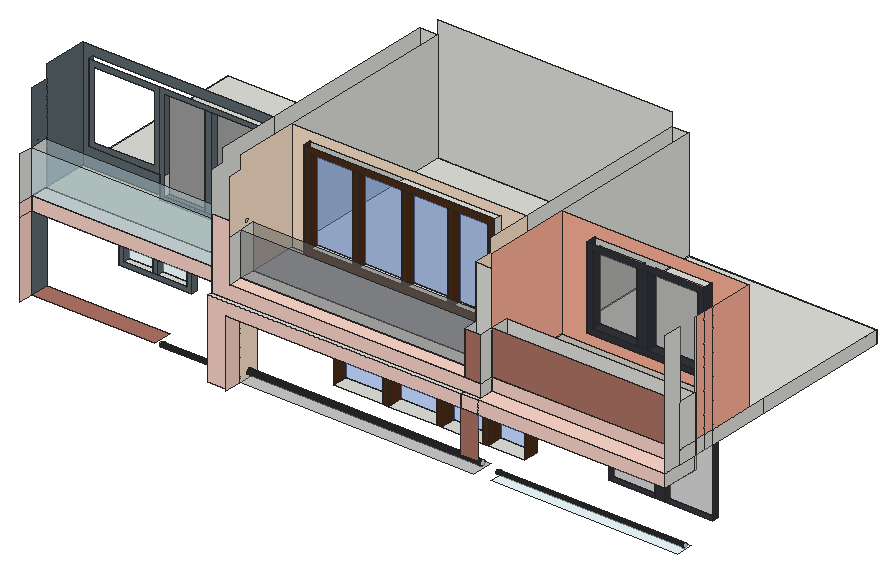
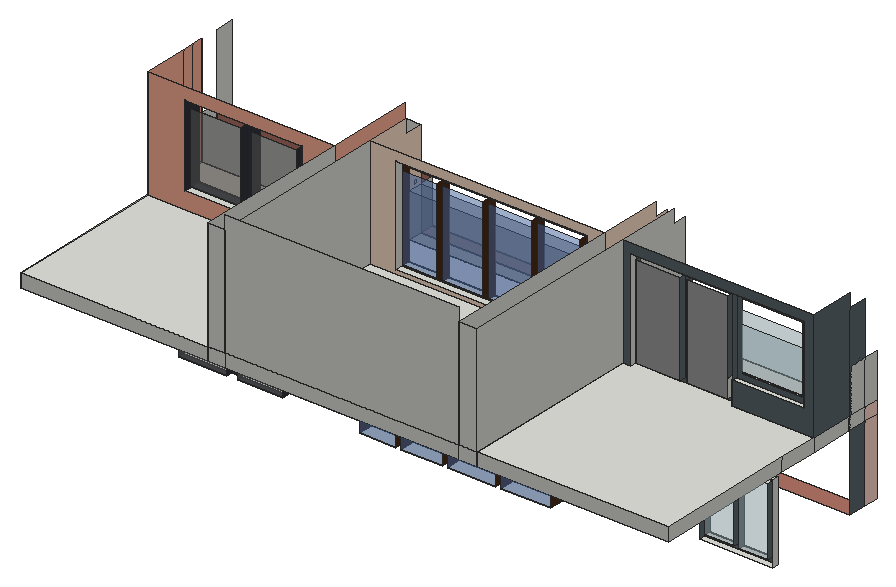
# SketchUp Ruby script. Lengths in inches.
U = 1.inch
M = Sketchup.active_model
def pt(a) = Geom::Point3d.new(a.map { |v| v * U })
def face(e, loops, mat)
  f = e.add_face(loops[0].map { |a| pt(a) })
  loops[1..].each { |l| e.add_face(l.map { |a| pt(a) }).erase! }
  f.material = f.back_material = mat if mat
  f
end
# faces: each face lists its corners as indices into pts; further lists are holes
def faces(e, pts, list, mat = nil) = list.each { |f| face(e, (f[0].is_a?(Array) ? f : [f]).map { |l| l.map { |i| pts[i] } }, mat) }
# xy, xz, yz: faces in a plane at the given z, y or x. An outline is a flat list of corners, or four numbers for a rectangle; further outlines are holes
def ring(l) = l.size == 4 ? [[l[0], l[1]], [l[2], l[1]], [l[2], l[3]], [l[0], l[3]]] : l.each_slice(2).to_a
def flat(e, list, mat, &to3) = list.each { |f| face(e, (f[0].is_a?(Array) ? f : [f]).map { |l| ring(l).map { |u, v| to3.(u, v) } }, mat) }
def xy(e, z, list, mat = nil) = flat(e, list, mat) { |x, y| [x, y, z] }
def xz(e, y, list, mat = nil) = flat(e, list, mat) { |x, z| [x, y, z] }
def yz(e, x, list, mat = nil) = flat(e, list, mat) { |y, z| [x, y, z] }
def lines(e, pts, list) = list.each { |a, b| e.add_line(pt(pts[a]), pt(pts[b])) }
# prism: a flat outline (further loops are holes) pulled along v
def prism(e, loops, v, mat = nil)
  f = face(e, loops, mat); d = Geom::Vector3d.new(v.map { |x| x * U })
  f.pushpull(f.normal.samedirection?(d) ? d.length : -d.length)
end
def box(e, o, s, mat = nil) = prism(e, [[o, [o[0] + s[0], o[1], o[2]], [o[0] + s[0], o[1] + s[1], o[2]], [o[0], o[1] + s[1], o[2]]]], [0, 0, s[2]], mat)
def at(x, y, z, deg = 0) = Geom::Transformation.translation(pt([x, y, z])) * Geom::Transformation.rotation(ORIGIN, Z_AXIS, deg.degrees)
def axes(o, x, y, z) = Geom::Transformation.new([*x, 0, *y, 0, *z, 0, *pt(o).to_a, 1])
def part(name) = M.definitions.add(name)
# library, detail: a bought-in or finely detailed component or shape, given as its bounding box
def library(name, o, s) = part(name).tap { |d| box(d.entities, o, s) }
def detail(e, o, s) = box(e.add_group.entities, o, s)
def put(e, d, t, mat = nil) = e.add_instance(d, t).tap { |i| i.material = mat if mat }
def group(e, t, mat = nil) = e.add_group.tap { |g| g.transformation = t; g.material = mat if mat }.entities
root = M.entities
M.materials.add("[Blinds Vertical Stripe Gray]").color = [160, 160, 160]
M.materials.add("[Color B01]").color = [255, 216, 204]
M.materials.add("[Color B02]").color = [255, 178, 153]
M.materials.add("[Color C01]").color = [255, 229, 204]
M.materials.add("[Field Rectangle Tile]").color = [196, 189, 179]
M.materials.add("[Field Square Tile]").color = [217, 201, 169]
M.materials.add("[Formica Graystone]").color = [149, 146, 135]
M.materials.add("[Formica Laminate Dark]").color = [50, 53, 60]
M.materials.add("[Formica Speckled Grey]").color = [94, 105, 111]
M.materials.add("[Marble Carrara Floor Tile]").color = [204, 208, 219]
M.materials.add("[Stone Flagstone Ashlar]").color = [175, 116, 102]
M.materials.add("[Stone Flagstone Ashlar]1").color = [175, 116, 102]
M.materials.add("[Terrazzo Tile Light]").color = [219, 217, 210]
M.materials.add("[Translucent Glass Blue]").color = [100, 149, 237]
M.materials["[Translucent Glass Blue]"].alpha = 0.5
M.materials.add("[Translucent Glass Gray]").color = [128, 128, 128]
M.materials["[Translucent Glass Gray]"].alpha = 0.5
M.materials.add("[Translucent Glass Safety]").color = [204, 235, 244]
M.materials["[Translucent Glass Safety]"].alpha = 0.5
M.materials.add("[Wood Veneer 01]").color = [76, 44, 23]
xy(root,776.18,[[1324.98,1141.09,1459.45,1182.72],[1473.64,1141.09,1605.14,1182.72],[1619.33,1141.09,1732.89,1182.72],[1747.08,1141.09,1847.2,1182.72]])
xy(root,789.44,[[2056.09,1166.78,2180.58,1182.72],[2208.79,1166.78,2341.44,1182.72]],"[Formica Laminate Dark]")
xy(root,844.43,[[715.78,1166.28,917.47,1182.72]])
xy(root,858.1,[[729.45,1166.28,809.37,1182.72],[823.58,1166.28,903.8,1182.72]])
xy(root,868.4375,[[1131.83,916.51,1132.91,916.65,1133.92,917.07,1134.79,917.73,1135.46,918.6,1135.875,919.61,1136.02,920.69,1135.875,921.78,1135.46,922.79,1134.79,923.65,1133.92,924.32,1132.91,924.74,1131.83,924.88,1130.75,924.74,1129.74,924.32,1128.87,923.65,1128.2,922.79,1127.79,921.78,1127.64,920.69,1127.79,919.61,1128.2,918.6,1128.87,917.73,1129.74,917.07,1130.75,916.65]])
xy(root,868.4375,[[1263.92,894.5,1905.54,954.56]],"[Translucent Glass Gray]")
xy(root,868.4375,[[1950.59,894.5,2463.34,942.43]],"[Translucent Glass Safety]")
xy(root,868.5625,[[1101.58,916.51,1102.66,916.65,1103.67,917.07,1104.54,917.73,1105.21,918.6,1105.625,919.61,1105.77,920.69,1105.625,921.78,1105.21,922.79,1104.54,923.65,1103.67,924.32,1102.66,924.74,1101.58,924.88,1100.5,924.74,1099.49,924.32,1098.62,923.65,1097.95,922.79,1097.54,921.78,1097.39,920.69,1097.54,919.61,1097.95,918.6,1098.62,917.73,1099.49,917.07,1100.5,916.65]])
xy(root,868.875,[[1167.14,916.51,1168.23,916.65,1169.24,917.07,1170.1,917.73,1170.77,918.6,1171.1875,919.61,1171.33,920.69,1171.1875,921.78,1170.77,922.79,1170.1,923.65,1169.24,924.32,1168.23,924.74,1167.14,924.88,1166.06,924.74,1165.05,924.32,1164.18,923.65,1163.52,922.79,1163.1,921.78,1162.96,920.69,1163.1,919.61,1163.52,918.6,1164.18,917.73,1165.05,917.07,1166.06,916.65]])
xy(root,869.875,[[1198.52,916.51,1199.6,916.65,1200.61,917.07,1201.48,917.73,1202.14,918.6,1202.5625,919.61,1202.71,920.69,1202.5625,921.78,1202.14,922.79,1201.48,923.65,1200.61,924.32,1199.6,924.74,1198.52,924.88,1197.43,924.74,1196.42,924.32,1195.56,923.65,1194.89,922.79,1194.47,921.78,1194.33,920.69,1194.47,919.61,1194.89,918.6,1195.56,917.73,1196.42,917.07,1197.43,916.65]])
xy(root,871.18,[[1070.77,916.51,1071.85,916.65,1072.86,917.07,1073.55,917.6,1067.98,917.6,1068.67,917.07,1069.68,916.65],[1067.98,917.6,1073.55,917.6,1073.73,917.73,1074.39,918.6,1074.8125,919.61,1074.96,920.69,1074.8125,921.78,1074.39,922.79,1073.73,923.65,1072.86,924.32,1071.85,924.74,1070.77,924.88,1069.68,924.74,1068.67,924.32,1067.81,923.65,1067.14,922.79,1066.72,921.78,1066.58,920.69,1066.72,919.61,1067.14,918.6,1067.81,917.73]])
xy(root,871.5625,[[1041.89,916.51,1042.98,916.65,1043.99,917.07,1044.85,917.73,1045.52,918.6,1045.9375,919.61,1046.08,920.69,1045.9375,921.78,1045.52,922.79,1044.85,923.65,1043.99,924.32,1042.98,924.74,1041.89,924.88,1040.81,924.74,1039.8,924.32,1038.93,923.65,1038.27,922.79,1037.85,921.78,1037.71,920.69,1037.85,919.61,1038.27,918.6,1038.93,917.73,1039.8,917.07,1040.81,916.65]])
xy(root,880,[[691.11,899.87,1027.33,950.43]],"[Stone Flagstone Ashlar]")
xy(root,1043.49,[[2056.09,1166.78,2180.58,1182.72],[2208.79,1166.78,2341.44,1182.72]],"[Formica Laminate Dark]")
xy(root,1045.08,[[1324.98,1141.09,1459.45,1182.72],[1473.64,1141.09,1605.14,1182.72],[1619.33,1141.09,1732.89,1182.72],[1747.08,1141.09,1847.2,1182.72]],"[Wood Veneer 01]")
xy(root,1045.24,[[729.45,1166.28,809.37,1182.72],[823.58,1166.28,903.8,1182.72]])
xy(root,1051.41,[[1905.54,849.3125,1905.54,894.5,1263.92,894.5,1263.92,954.56,2463.34,954.56,2463.34,849.3125]],"[Color B02]")
xy(root,1051.41,[[1263.92,849.3125,1905.54,894.5]],"[Color C01]")
xy(root,1058.91,[[715.78,1166.28,917.47,1182.72]])
xy(root,1058.91,[[1009.02,1166.28,1195.59,1182.72]],"[Formica Speckled Grey]")
xy(root,1059.16,[[1310.9,1141.09,1861.28,1182.72]])
xy(root,1063.34,[[2036.23,1166.78,2361.3,1182.72]])
xy(root,1086.8125,[[1214.63,849.3125,1905.54,861.43],[1905.54,849.3125,1950.59,861.43],[1214.63,861.43,1263.92,894.5],[1263.92,861.43,1905.54,894.5],[1905.54,861.43,1950.59,954.56],
  [1214.63,894.5,1263.92,1182.72],[1263.92,894.5,1905.54,954.56],[1950.59,899.87,2463.34,954.56],[1905.54,954.56,1950.59,1571.68],[691.11,1182.72,1214.63,1571.68],
  [1214.63,1182.72,1263.92,1571.68],[1263.92,1182.72,1905.54,1571.68],[1950.59,1182.72,2463.34,1571.68]])
xy(root,1086.8125,[[1950.59,849.3125,2463.34,899.87]],"[Color B01]")
xy(root,1086.8125,[[1950.59,954.56,2463.34,1182.72]],"[Color B02]")
xy(root,1086.8125,[[1263.92,954.56,1905.54,1182.72]],"[Color C01]")
xy(root,1086.8125,[[691.11,899.87,1214.63,1182.72]],"[Terrazzo Tile Light]")
xy(root,1122.8125,[[1905.54,861.43,1950.59,899.87],[691.11,899.87,1214.63,947.14],[1263.92,899.87,1905.54,941.11],[1905.54,899.87,1950.59,1571.68],[1950.59,899.87,2463.34,950.43],
  [915.76,1058.36,1191.39,1058.36,1191.39,1074.11,1214.63,1074.11,1214.63,1571.68,691.11,1571.68,691.11,1074.11,915.76,1074.11],[1263.92,1074.11,1905.54,1571.68],[1950.59,1136.84,2463.34,1571.68]])
xy(root,1122.8125,[[1263.92,861.43,1905.54,899.87]],"[Color B01]")
xy(root,1122.8125,[[1950.59,950.43,2463.34,1136.84]],"[Field Rectangle Tile]")
xy(root,1122.8125,[[691.11,947.14,1214.63,947.14,1214.63,1074.11,1191.39,1074.11,1191.39,1058.36,915.76,1058.36,915.76,1074.11,691.11,1074.11]],"[Field Square Tile]")
xy(root,1122.8125,[[1263.92,941.11,1905.54,1074.11]],"[Marble Carrara Floor Tile]")
xy(root,1132.49,[[1313.52,1053.48,1834.21,1074.11]])
xy(root,1134.65,[[927.6,1058.36,1038.4,1074.11],[1057.92,1058.36,1179.55,1074.11]],"[Formica Speckled Grey]")
xy(root,1150.02,[[1331.05,1053.48,1447.61,1074.11],[1463.69,1053.48,1579.86,1074.11],[1595.94,1053.48,1706.36,1074.11],[1722.44,1053.48,1816.68,1074.11]])
xy(root,1167.86,[[2040.39,1110.15,2360.64,1136.84]])
xy(root,1183.82,[[2056.35,1110.15,2178.28,1136.84],[2208.51,1110.15,2344.68,1136.84]],"[Formica Laminate Dark]")
xy(root,1184.88,[[719.95,1058.36,915.76,1074.11]])
xz(root,849.3125,[[1214.63,872.4,1263.92,872.4,1263.92,1051.41,1905.54,1051.41,1905.54,1086.8125,1214.63,1086.8125],[1905.54,1051.41,1950.59,1086.8125],[1950.59,1051.41,2463.34,1086.8125]],"[Color B01]")
xz(root,849.3125,[[1905.54,937.95,1950.59,1051.41]],"[Stone Flagstone Ashlar]1")
xz(root,861.43,[[1214.63,1086.8125,1950.59,1086.8125,1950.59,1122.8125,1263.92,1122.8125,1263.92,1280.46,1214.63,1280.46]],"[Color B01]")
xz(root,861.43,[[1905.54,1122.8125,1950.59,1241.6875]],"[Stone Flagstone Ashlar]1")
xz(root,899.87,[[1905.54,1122.8125,1950.59,1387.1]])
xz(root,899.87,[[691.11,1086.8125,1214.63,1122.8125],[1950.59,1086.8125,2463.34,1122.8125]],"[Color B01]")
xz(root,899.87,[[1950.59,1122.8125,2463.34,1241.6875]],"[Stone Flagstone Ashlar]")
xz(root,899.87,[[1263.92,1122.8125,1905.54,1241.6875]],"[Translucent Glass Gray]")
xz(root,899.87,[[691.11,1122.8125,1214.63,1241.6875]],"[Translucent Glass Safety]")
xz(root,941.11,[[1263.92,1122.8125,1905.54,1241.6875]],"[Translucent Glass Gray]")
xz(root,947.14,[[691.11,1122.8125,1214.63,1241.6875]],"[Translucent Glass Safety]")
xz(root,950.43,[[1950.59,1122.8125,2463.34,1241.6875]])
xz(root,954.56,[[1263.92,1051.41,2463.34,1086.8125]])
xz(root,1053.48,[[[1313.52,1132.49,1834.21,1400.05],[1331.05,1150.02,1816.68,1382.52]],[1447.61,1150.02,1463.69,1382.52],[1579.86,1150.02,1595.94,1382.52],[1706.36,1150.02,1722.44,1382.52]],"[Wood Veneer 01]")
xz(root,1058.36,[[[915.76,1122.8125,1191.39,1398.44],[927.6,1134.65,1179.55,1386.6]],[1038.4,1134.65,1057.92,1386.6],[[719.95,1184.88,915.76,1398.44],[734.47,1199.4,901.24,1383.92]]],"[Formica Speckled Grey]")
xz(root,1074.11,[[927.6,1134.65,1038.4,1386.6],[1057.92,1134.65,1179.55,1386.6]],"[Blinds Vertical Stripe Gray]")
xz(root,1074.11,[[[1263.92,1122.8125,1905.54,1424.1875],[1313.52,1132.49,1834.21,1400.05]]],"[Color C01]")
xz(root,1074.11,[[691.11,1122.8125,915.76,1122.8125,915.76,1184.88,719.95,1184.88,719.95,1398.44,1191.39,1398.44,1191.39,1122.8125,1214.63,1122.8125,1214.63,1424.1875,691.11,1424.1875]],"[Formica Speckled Grey]")
xz(root,1074.11,[[1331.05,1150.02,1447.61,1382.52],[1463.69,1150.02,1579.86,1382.52],[1595.94,1150.02,1706.36,1382.52],[1722.44,1150.02,1816.68,1382.52]],"[Translucent Glass Blue]")
xz(root,1110.15,[[[2040.39,1167.86,2360.64,1392.23],[2056.35,1183.82,2344.68,1376.27]],[2178.28,1183.82,2208.51,1376.27]],"[Formica Laminate Dark]")
xz(root,1136.84,[[[1950.59,1122.8125,2463.34,1424.1875],[2040.39,1167.86,2360.64,1392.23]]],"[Color B02]")
xz(root,1136.84,[[2056.35,1183.82,2178.28,1376.27],[2208.51,1183.82,2344.68,1376.27]],"[Translucent Glass Gray]")
xz(root,1141.09,[[1459.45,776.18,1473.64,1045.08],[1605.14,776.18,1619.33,1045.08],[1732.89,776.18,1747.08,1045.08]],"[Wood Veneer 01]")
xz(root,1166.28,[[[715.78,844.43,917.47,1058.91],[729.45,858.1,903.8,1045.24]],[809.37,858.1,823.58,1045.24],[1009.02,1033.9,1195.59,1058.91]],"[Formica Speckled Grey]")
xz(root,1166.78,[[2180.58,789.44,2208.79,1043.49]],"[Formica Laminate Dark]")
xz(root,1182.72,[[1324.98,776.18,1459.45,1045.08],[1473.64,776.18,1605.14,1045.08],[1619.33,776.18,1732.89,1045.08],[1747.08,776.18,1847.2,1045.08]],"[Translucent Glass Blue]")
xz(root,1182.72,[[2056.09,789.44,2180.58,1043.49],[2208.79,789.44,2341.44,1043.49]],"[Translucent Glass Gray]")
xz(root,1182.72,[[729.45,858.1,809.37,1045.24],[823.58,858.1,903.8,1045.24]],"[Translucent Glass Safety]")
xz(root,1571.68,[[691.11,1086.8125,1214.63,1122.8125],[1214.63,1086.8125,1263.92,1122.8125],[1263.92,1086.8125,1905.54,1122.8125],[1905.54,1086.8125,1950.59,1122.8125],[1950.59,1086.8125,2463.34,1122.8125],
  [1214.63,1122.8125,1263.92,1424.1875],[1263.92,1122.8125,1905.54,1460.1875],[1905.54,1122.8125,1950.59,1424.1875]])
yz(root,691.11,[[899.87,1086.8125,950.43,1122.8125],[950.43,1086.8125,954.56,1122.8125],[954.56,1086.8125,1074.11,1122.8125],[1074.11,1086.8125,1182.72,1122.8125],[1182.72,1086.8125,1571.68,1122.8125],
  [861.43,1122.8125,899.87,1241.6875],[899.87,1122.8125,947.14,1241.6875]])
yz(root,691.11,[[861.43,880,899.87,1086.8125],[861.43,1086.8125,899.87,1122.8125]],"[Color B01]")
yz(root,691.11,[[899.87,880,950.43,1086.8125],[[947.14,1122.8125,950.43,1122.8125,950.43,1387.1,899.87,1387.1,899.87,1241.6875,947.14,1241.6875],[922.41,1246.62,921.41,1246.65,920.46,1246.93,919.61,1247.46,918.93,1248.18,918.45,1249.05,918.22,1250.02,918.25,1251.02,918.54,1251.97,919.06,1252.82,919.78,1253.5,920.66,1253.98,921.625,1254.21,922.62,1254.18,923.58,1253.89,924.42,1253.37,925.11,1252.65,925.58,1251.77,925.81,1250.8,925.78,1249.81,925.5,1248.85,924.97,1248.01,924.25,1247.32,923.375,1246.85]],[950.43,1122.8125,1074.11,1424.1875]],"[Formica Speckled Grey]")
yz(root,715.78,[[1166.28,844.43,1182.72,1058.91]])
yz(root,719.95,[[1058.36,1184.88,1074.11,1398.44]],"[Formica Speckled Grey]")
yz(root,729.45,[[1166.28,858.1,1182.72,1045.24]],"[Formica Speckled Grey]")
yz(root,809.37,[[1166.28,858.1,1182.72,1045.24]],"[Formica Speckled Grey]")
yz(root,823.58,[[1166.28,858.1,1182.72,1045.24]],"[Formica Speckled Grey]")
yz(root,903.8,[[1166.28,858.1,1182.72,1045.24]],"[Formica Speckled Grey]")
yz(root,915.76,[[1058.36,1122.8125,1074.11,1184.88]])
yz(root,917.47,[[1166.28,844.43,1182.72,1058.91]],"[Formica Speckled Grey]")
yz(root,927.6,[[1058.36,1134.65,1074.11,1184.88]])
yz(root,927.6,[[1058.36,1184.88,1074.11,1386.6]],"[Formica Speckled Grey]")
yz(root,1009.02,[[1166.28,1033.9,1182.72,1058.91]],"[Formica Speckled Grey]")
yz(root,1027.33,[[922.52,862.65,921.05,862.84,919.68,863.41,918.5,864.32,917.6,865.49,917.03,866.87,916.84,868.34,917.03,869.81,917.6,871.18,918.5,872.36,919.68,873.26,921.05,873.83,922.52,874.02,923.99,873.83,925.37,873.26,926.54,872.36,927.45,871.18,928.02,869.81,928.21,868.34,928.02,866.87,927.45,865.49,926.54,864.32,925.37,863.41,923.99,862.84]])
yz(root,1038.4,[[1058.36,1134.65,1074.11,1386.6]],"[Formica Speckled Grey]")
yz(root,1057.92,[[1058.36,1134.65,1074.11,1386.6]],"[Formica Speckled Grey]")
yz(root,1179.55,[[1058.36,1134.65,1074.11,1386.6]],"[Formica Speckled Grey]")
yz(root,1191.39,[[1058.36,1122.8125,1074.11,1398.44]])
yz(root,1195.59,[[1166.28,1033.9,1182.72,1058.91]],"[Formica Speckled Grey]")
yz(root,1214.63,[[899.87,1086.8125,1571.68,1122.8125],[[947.14,1122.8125,947.14,1241.6875,861.43,1241.6875,861.43,1387.1,899.87,1387.1,899.87,1424.1875,1074.11,1424.1875,1074.11,1122.8125],[922.41,1246.62,923.375,1246.85,924.25,1247.32,924.97,1248.01,925.5,1248.85,925.78,1249.81,925.81,1250.8,925.58,1251.77,925.11,1252.65,924.42,1253.37,923.58,1253.89,922.62,1254.18,921.625,1254.21,920.66,1253.98,919.78,1253.5,919.06,1252.82,918.54,1251.97,918.25,1251.02,918.22,1250.02,918.45,1249.05,918.93,1248.18,919.61,1247.46,920.46,1246.93,921.41,1246.65]],[899.87,1122.8125,947.14,1241.6875],[1074.11,1122.8125,1571.68,1424.1875]])
yz(root,1214.63,[[861.43,1086.8125,899.87,1122.8125],[861.43,1122.8125,899.87,1241.6875]],"[Color B01]")
yz(root,1263.92,[[861.43,1122.8125,899.87,1241.6875],[899.87,1122.8125,941.11,1241.6875],[1074.11,1122.8125,1571.68,1424.1875]])
yz(root,1263.92,[[849.3125,868.4375,894.5,1051.41]],"[Color B01]")
yz(root,1263.92,[[[894.5,868.4375,954.56,1051.41],[923.73,877.96,922,878.18,920.39,878.85,919,879.91,917.94,881.3,917.27,882.91,917.04,884.64,917.27,886.375,917.94,887.99,919,889.37,920.39,890.43,922,891.1,923.73,891.33,925.46,891.1,927.08,890.43,928.46,889.37,929.52,887.99,930.19,886.375,930.42,884.64,930.19,882.91,929.52,881.3,928.46,879.91,927.08,878.85,925.46,878.18]],[[941.11,1122.8125,1074.11,1122.8125,1074.11,1424.1875,899.87,1424.1875,899.87,1387.1,861.43,1387.1,861.43,1241.6875,941.11,1241.6875],[918.53,1249.2,916.83,1249.42,915.25,1250.08,913.89,1251.12,912.85,1252.48,912.19,1254.0625,911.97,1255.76,912.19,1257.46,912.85,1259.04,913.89,1260.4,915.25,1261.45,916.83,1262.1,918.53,1262.33,920.23,1262.1,921.8125,1261.45,923.17,1260.4,924.21,1259.04,924.87,1257.46,925.09,1255.76,924.87,1254.0625,924.21,1252.48,923.17,1251.12,921.8125,1250.08,920.23,1249.42]]],"[Color C01]")
yz(root,1313.52,[[1053.48,1132.49,1074.11,1400.05]],"[Wood Veneer 01]")
yz(root,1324.98,[[1141.09,776.18,1182.72,1045.08]],"[Wood Veneer 01]")
yz(root,1331.05,[[1053.48,1150.02,1074.11,1382.52]],"[Wood Veneer 01]")
yz(root,1447.61,[[1053.48,1150.02,1074.11,1382.52]],"[Wood Veneer 01]")
yz(root,1459.45,[[1141.09,776.18,1182.72,1045.08]],"[Wood Veneer 01]")
yz(root,1463.69,[[1053.48,1150.02,1074.11,1382.52]],"[Wood Veneer 01]")
yz(root,1473.64,[[1141.09,776.18,1182.72,1045.08]],"[Wood Veneer 01]")
yz(root,1579.86,[[1053.48,1150.02,1074.11,1382.52]],"[Wood Veneer 01]")
yz(root,1595.94,[[1053.48,1150.02,1074.11,1382.52]],"[Wood Veneer 01]")
yz(root,1605.14,[[1141.09,776.18,1182.72,1045.08]],"[Wood Veneer 01]")
yz(root,1619.33,[[1141.09,776.18,1182.72,1045.08]],"[Wood Veneer 01]")
yz(root,1706.36,[[1053.48,1150.02,1074.11,1382.52]],"[Wood Veneer 01]")
yz(root,1722.44,[[1053.48,1150.02,1074.11,1382.52]],"[Wood Veneer 01]")
yz(root,1732.89,[[1141.09,776.18,1182.72,1045.08]],"[Wood Veneer 01]")
yz(root,1747.08,[[1141.09,776.18,1182.72,1045.08]],"[Wood Veneer 01]")
yz(root,1816.68,[[1053.48,1150.02,1074.11,1382.52]],"[Wood Veneer 01]")
yz(root,1834.21,[[1053.48,1132.49,1074.11,1400.05]])
yz(root,1847.2,[[1141.09,776.18,1182.72,1045.08]],"[Wood Veneer 01]")
yz(root,1905.54,[[923.73,877.96,925.46,878.18,927.08,878.85,928.46,879.91,929.52,881.3,930.19,882.91,930.42,884.64,930.19,886.375,929.52,887.99,928.46,889.37,927.08,890.43,925.46,891.1,923.73,891.33,922,891.1,920.39,890.43,919,889.37,917.94,887.99,917.27,886.375,917.04,884.64,917.27,882.91,917.94,881.3,919,879.91,920.39,878.85,922,878.18],[849.3125,1051.41,894.5,1086.8125],[861.43,1122.8125,899.87,1241.6875],[899.87,1122.8125,941.11,1241.6875],[1074.11,1122.8125,1571.68,1424.1875]])
yz(root,1905.54,[[[941.11,1122.8125,941.11,1241.6875,899.87,1241.6875,899.87,1387.1,950.43,1387.1,950.43,1424.1875,1074.11,1424.1875,1074.11,1122.8125],[918.53,1249.2,920.23,1249.42,921.8125,1250.08,923.17,1251.12,924.21,1252.48,924.87,1254.0625,925.09,1255.76,924.87,1257.46,924.21,1259.04,923.17,1260.4,921.8125,1261.45,920.23,1262.1,918.53,1262.33,916.83,1262.1,915.25,1261.45,913.89,1260.4,912.85,1259.04,912.19,1257.46,911.97,1255.76,912.19,1254.0625,912.85,1252.48,913.89,1251.12,915.25,1250.08,916.83,1249.42]]],"[Color C01]")
yz(root,1950.59,[[861.43,1086.8125,899.87,1122.8125],[899.87,1086.8125,1571.68,1122.8125],[861.43,1122.8125,899.87,1241.6875],[899.87,1122.8125,950.43,1241.6875],[1136.84,1122.8125,1571.68,1424.1875]])
yz(root,1950.59,[[950.43,1122.8125,1136.84,1122.8125,1136.84,1424.1875,899.87,1424.1875,899.87,1241.6875,950.43,1241.6875]],"[Color B02]")
yz(root,2040.39,[[1110.15,1167.86,1136.84,1392.23]],"[Formica Laminate Dark]")
yz(root,2056.09,[[1166.78,789.44,1182.72,1043.49]],"[Formica Laminate Dark]")
yz(root,2056.35,[[1110.15,1183.82,1136.84,1376.27]],"[Formica Laminate Dark]")
yz(root,2178.28,[[1110.15,1183.82,1136.84,1376.27]],"[Formica Laminate Dark]")
yz(root,2180.58,[[1166.78,789.44,1182.72,1043.49]],"[Formica Laminate Dark]")
yz(root,2208.51,[[1110.15,1183.82,1136.84,1376.27]],"[Formica Laminate Dark]")
yz(root,2208.79,[[1166.78,789.44,1182.72,1043.49]],"[Formica Laminate Dark]")
yz(root,2341.44,[[1166.78,789.44,1182.72,1043.49]],"[Formica Laminate Dark]")
yz(root,2344.68,[[1110.15,1183.82,1136.84,1376.27]],"[Formica Laminate Dark]")
yz(root,2360.64,[[1110.15,1167.86,1136.84,1392.23]],"[Formica Laminate Dark]")
yz(root,2463.34,[[918.47,876.58,919.74,876.75,920.93,877.24,921.96,878.03,922.74,879.05,923.23,880.24,923.4,881.52,923.23,882.8,922.74,883.99,921.96,885.01,920.93,885.8,919.74,886.29,918.47,886.46,917.1875,886.29,916,885.8,914.97,885.01,914.1875,883.99,913.7,882.8,913.53,881.52,913.7,880.24,914.1875,879.05,914.97,878.03,916,877.24,917.1875,876.75],[849.3125,1051.41,950.43,1086.8125],[950.43,1051.41,954.56,1086.8125],[849.3125,1086.8125,899.87,1424.1875],[899.87,1086.8125,950.43,1122.8125],
  [950.43,1086.8125,954.56,1122.8125],[954.56,1086.8125,983.36,1122.8125],[983.36,1086.8125,1012.29,1122.8125],[1012.29,1086.8125,1182.72,1122.8125],[1182.72,1086.8125,1571.68,1122.8125],
  [899.87,1122.8125,950.43,1241.6875],[950.43,1122.8125,954.56,1424.1875]])
yz(root,2463.34,[[954.56,1122.8125,983.36,1424.1875],[983.36,1122.8125,1012.29,1424.1875],[1012.29,1122.8125,1136.84,1424.1875]],"[Color B02]")
p = [[1027.33,921.05,862.84],[1027.33,922.52,862.65],[1214.63,922.52,862.65],[1214.63,921.05,862.84],[1027.33,923.99,862.84],[1214.63,923.99,862.84],
  [1027.33,919.68,863.41],[1214.63,919.68,863.41],[1027.33,925.37,863.41],[1214.63,925.37,863.41],[1027.33,918.5,864.32],[1214.63,918.5,864.32],
  [1027.33,926.54,864.32],[1214.63,926.54,864.32],[1027.33,917.6,865.49],[1214.63,917.6,865.49],[1027.33,927.45,865.49],[1214.63,927.45,865.49],
  [1027.33,917.03,866.87],[1214.63,917.03,866.87],[1027.33,928.02,866.87],[1214.63,928.02,866.87],[1027.33,916.84,868.34],[1214.63,916.84,868.34],
  [1027.33,928.21,868.34],[1214.63,928.21,868.34],[1027.33,917.03,869.81],[1214.63,917.03,869.81],[1027.33,928.02,869.81],[1214.63,928.02,869.81],
  [1027.33,917.6,871.18],[1214.63,917.6,871.18],[1073.55,917.6,871.18],[1067.98,917.6,871.18],[1027.33,927.45,871.18],[1214.63,927.45,871.18],
  [1027.33,918.5,872.36],[1214.63,918.5,872.36],[1027.33,926.54,872.36],[1214.63,926.54,872.36],[1027.33,919.68,873.26],[1214.63,919.68,873.26],
  [1027.33,925.37,873.26],[1214.63,925.37,873.26],[1027.33,921.05,873.83],[1214.63,921.05,873.83],[1027.33,923.99,873.83],[1214.63,923.99,873.83],
  [1027.33,922.52,874.02],[1214.63,922.52,874.02],[2463.34,918.47,876.58],[2463.34,917.1875,876.75],[1950.59,917.1875,876.75],[1950.59,918.47,876.58],
  [2463.34,919.74,876.75],[1950.59,919.74,876.75],[2463.34,916,877.24],[1950.59,916,877.24],[2463.34,920.93,877.24],[1950.59,920.93,877.24],
  [2463.34,914.97,878.03],[1950.59,914.97,878.03],[2463.34,921.96,878.03],[1950.59,921.96,878.03],[2463.34,914.1875,879.05],[1950.59,914.1875,879.05],
  [1905.54,923.73,877.96],[1905.54,922,878.18],[1263.92,922,878.18],[1263.92,923.73,877.96],[2463.34,922.74,879.05],[1950.59,922.74,879.05],
  [1905.54,925.46,878.18],[1263.92,925.46,878.18],[1905.54,920.39,878.85],[1263.92,920.39,878.85],[1905.54,927.08,878.85],[1263.92,927.08,878.85],
  [1905.54,919,879.91],[1263.92,919,879.91],[1905.54,928.46,879.91],[1263.92,928.46,879.91],[2463.34,913.7,880.24],[1950.59,913.7,880.24],
  [2463.34,923.23,880.24],[1950.59,923.23,880.24],[1905.54,917.94,881.3],[1263.92,917.94,881.3],[1905.54,929.52,881.3],[1263.92,929.52,881.3],
  [2463.34,913.53,881.52],[1950.59,913.53,881.52],[2463.34,923.4,881.52],[1950.59,923.4,881.52],[1905.54,917.27,882.91],[1263.92,917.27,882.91],
  [1905.54,930.19,882.91],[1263.92,930.19,882.91],[2463.34,913.7,882.8],[1950.59,913.7,882.8],[2463.34,923.23,882.8],[1950.59,923.23,882.8],
  [2463.34,914.1875,883.99],[1950.59,914.1875,883.99],[2463.34,922.74,883.99],[1950.59,922.74,883.99],[1905.54,917.04,884.64],[1263.92,917.04,884.64],
  [1905.54,930.42,884.64],[1263.92,930.42,884.64],[2463.34,914.97,885.01],[1950.59,914.97,885.01],[2463.34,921.96,885.01],[1950.59,921.96,885.01],
  [1905.54,917.27,886.375],[1263.92,917.27,886.375],[1905.54,930.19,886.375],[1263.92,930.19,886.375],[2463.34,916,885.8],[1950.59,916,885.8],
  [2463.34,920.93,885.8],[1950.59,920.93,885.8],[2463.34,917.1875,886.29],[1950.59,917.1875,886.29],[2463.34,919.74,886.29],[1950.59,919.74,886.29],
  [2463.34,918.47,886.46],[1950.59,918.47,886.46],[1905.54,917.94,887.99],[1263.92,917.94,887.99],[1905.54,929.52,887.99],[1263.92,929.52,887.99],
  [1905.54,919,889.37],[1263.92,919,889.37],[1905.54,928.46,889.37],[1263.92,928.46,889.37],[1905.54,920.39,890.43],[1263.92,920.39,890.43],
  [1905.54,927.08,890.43],[1263.92,927.08,890.43],[1905.54,922,891.1],[1263.92,922,891.1],[1905.54,925.46,891.1],[1263.92,925.46,891.1],
  [1905.54,923.73,891.33],[1263.92,923.73,891.33]]
faces(root,p,[[0,1,2,3],[1,4,5,2],[6,0,3,7],[4,8,9,5],[10,6,7,11],[8,12,13,9],[14,10,11,15],[12,16,17,13],
  [18,14,15,19],[16,20,21,17],[22,18,19,23],[20,24,25,21],[26,22,23,27],[24,28,29,25],[30,26,27,31,32,33],[28,34,35,29],
  [36,30,33,32,31,37],[34,38,39,35],[40,36,37,41],[38,42,43,39],[44,40,41,45],[42,46,47,43],[48,44,45,49],[46,48,49,47]],"[Formica Graystone]")
faces(root,p,[[50,51,52,53],[54,50,53,55],[51,56,57,52],[58,54,55,59],[56,60,61,57],[62,58,59,63],[60,64,65,61],[66,67,68,69],
  [70,62,63,71],[72,66,69,73],[67,74,75,68],[76,72,73,77],[74,78,79,75],[80,76,77,81],[64,82,83,65],[84,70,71,85],
  [78,86,87,79],[88,80,81,89],[82,90,91,83],[92,84,85,93],[86,94,95,87],[96,88,89,97],[90,98,99,91],[100,92,93,101],
  [98,102,103,99],[104,100,101,105],[94,106,107,95],[108,96,97,109],[102,110,111,103],[112,104,105,113],[106,114,115,107],[116,108,109,117],
  [110,118,119,111],[120,112,113,121],[118,122,123,119],[124,120,121,125],[122,126,127,123],[126,124,125,127],[114,128,129,115],[130,116,117,131],
  [128,132,133,129],[134,130,131,135],[132,136,137,133],[138,134,135,139],[136,140,141,137],[142,138,139,143],[140,144,145,141],[144,142,143,145]],"[Formica Laminate Dark]")
